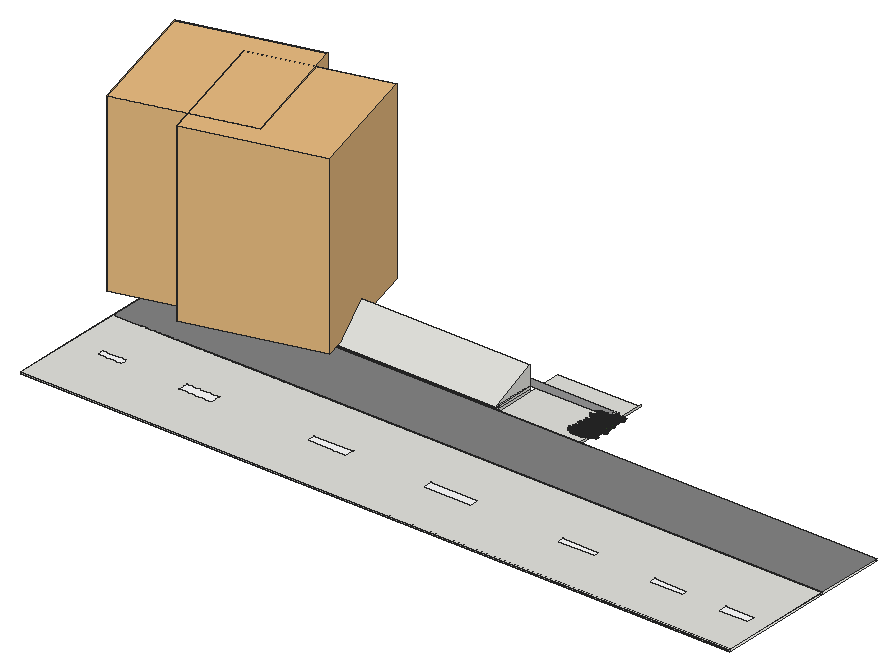
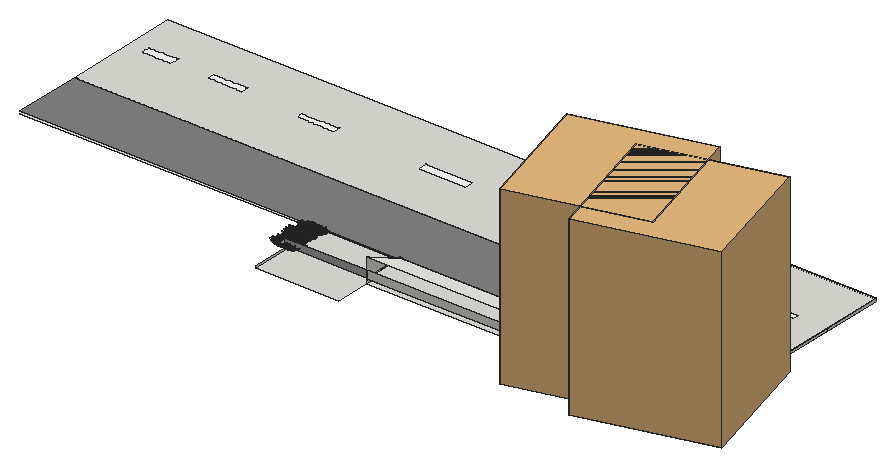
# SketchUp Ruby script. Lengths in inches.
U = 1.inch
M = Sketchup.active_model
def pt(a) = Geom::Point3d.new(a.map { |v| v * U })
def face(e, loops, mat)
  f = e.add_face(loops[0].map { |a| pt(a) })
  loops[1..].each { |l| e.add_face(l.map { |a| pt(a) }).erase! }
  f.material = f.back_material = mat if mat
  f
end
# faces: each face lists its corners as indices into pts; further lists are holes
def faces(e, pts, list, mat = nil) = list.each { |f| face(e, (f[0].is_a?(Array) ? f : [f]).map { |l| l.map { |i| pts[i] } }, mat) }
# xy, xz, yz: faces in a plane at the given z, y or x. An outline is a flat list of corners, or four numbers for a rectangle; further outlines are holes
def ring(l) = l.size == 4 ? [[l[0], l[1]], [l[2], l[1]], [l[2], l[3]], [l[0], l[3]]] : l.each_slice(2).to_a
def flat(e, list, mat, &to3) = list.each { |f| face(e, (f[0].is_a?(Array) ? f : [f]).map { |l| ring(l).map { |u, v| to3.(u, v) } }, mat) }
def xy(e, z, list, mat = nil) = flat(e, list, mat) { |x, y| [x, y, z] }
def xz(e, y, list, mat = nil) = flat(e, list, mat) { |x, z| [x, y, z] }
def yz(e, x, list, mat = nil) = flat(e, list, mat) { |y, z| [x, y, z] }
def lines(e, pts, list) = list.each { |a, b| e.add_line(pt(pts[a]), pt(pts[b])) }
# prism: a flat outline (further loops are holes) pulled along v
def prism(e, loops, v, mat = nil)
  f = face(e, loops, mat); d = Geom::Vector3d.new(v.map { |x| x * U })
  f.pushpull(f.normal.samedirection?(d) ? d.length : -d.length)
end
def box(e, o, s, mat = nil) = prism(e, [[o, [o[0] + s[0], o[1], o[2]], [o[0] + s[0], o[1] + s[1], o[2]], [o[0], o[1] + s[1], o[2]]]], [0, 0, s[2]], mat)
def at(x, y, z, deg = 0) = Geom::Transformation.translation(pt([x, y, z])) * Geom::Transformation.rotation(ORIGIN, Z_AXIS, deg.degrees)
def axes(o, x, y, z) = Geom::Transformation.new([*x, 0, *y, 0, *z, 0, *pt(o).to_a, 1])
def part(name) = M.definitions.add(name)
# library, detail: a bought-in or finely detailed component or shape, given as its bounding box
def library(name, o, s) = part(name).tap { |d| box(d.entities, o, s) }
def detail(e, o, s) = box(e.add_group.entities, o, s)
def put(e, d, t, mat = nil) = e.add_instance(d, t).tap { |i| i.material = mat if mat }
def group(e, t, mat = nil) = e.add_group.tap { |g| g.transformation = t; g.material = mat if mat }.entities
root = M.entities
M.materials.add("Color_3").color = [255, 255, 255]
M.materials.add("Material82").color = [68, 110, 58]
M.materials.add("Material83").color = [48, 90, 38]
M.materials.add("Material84").color = [68, 110, 48]
M.materials.add("Material85").color = [48, 90, 48]
M.materials.add("Material86").color = [58, 110, 58]
M.materials.add("Material87").color = [58, 90, 38]
M.materials.add("Material88").color = [68, 100, 58]
M.materials.add("Material89").color = [48, 100, 38]
M.materials.add("[Color M03]1").color = [170, 170, 170]
M.materials.add("[Tile Grey]1").color = [132, 132, 132]
c1 = library("Palm tree",[-4.09,-4.52,0],[193.52,193.51,258.93])
c2 = part("Palm+Tree")
put(c2.entities,c1,at(25.51,-21.81,0,15))
c3 = library("Group\#612",[0,0,0],[32.91,53.52,103.45])
c4 = part("Untitled (5)")
xy(c4.entities,0,[[[158.81,26.5625,306.06,993.3125],[226.57,518.17,239.57,583.92],[225.28,357.51,237.28,411.51],[222.61,182.28,236.36,226.53],[239.71,931.55,251.46,972.3],[233.64,703.93,242.14,755.18],[240.05,835.03,248.8,880.53],[222.04,66.5,231.29,100.5]]])
xy(c4.entities,0,[[222.04,66.5,231.29,100.5],[222.61,182.28,236.36,226.53],[225.28,357.51,237.28,411.51],[226.57,518.17,239.57,583.92],[233.64,703.93,242.14,755.18],
  [240.05,835.03,248.8,880.53],[239.71,931.55,251.46,972.3]],"Color_3")
c5 = part("grass00")
p = [[-0.6875,0.15,0],[-0.56,0.08,5.52],[-0.04,0.03,2.76],[0.48,-0.02,0],[0.35,-0.02,5.52],[-0.1,-0.14,5.52],
  [-0.12,0.65,8.37],[-0.42,0.65,8.37]]
faces(c5.entities,p,[[0,1,2,3],[3,2,4],[1,5,2],[5,4,2],[1,6,5],[4,5,6],[7,6,1]])
c6 = part("Group16\#1")
put(c6.entities,c5,axes([1.44,-0.61,-0.01],[0.05352,0.12609,0],[-0.10704,0.04543,0.07239],[0.06664,-0.02828,0.11628]),"Material85")
put(c6.entities,c5,axes([0.76,-0.15,-0.01],[0.04676,0.24062,0],[-0.23162,0.04501,0.06642],[0.0652,-0.01267,0.23595]),"Material82")
put(c6.entities,c5,axes([0.79,0.01,-0.01],[-0.00606,0.34651,0],[-0.34381,-0.00602,0.0432],[0.04319,0.00076,0.34386]))
put(c6.entities,c5,axes([1,0.23,-0.01],[-0.07192,0.31144,0],[-0.28722,-0.06632,0.1236],[0.12043,0.02781,0.29478]),"Material84")
put(c6.entities,c5,axes([1.66,0.77,-0.01],[-0.13828,0.29651,0],[-0.21551,-0.1005,0.22471],[0.20365,0.09498,0.23779]),"Material89")
put(c6.entities,c5,axes([0.6875,0.52,-0.01],[-0.18126,0.24051,0],[-0.22746,-0.17142,0.09788],[0.07817,0.05891,0.28481]),"Material84")
put(c6.entities,c5,axes([0.68,0.78,-0.01],[-0.215,0.18688,0],[-0.12385,-0.14248,0.21334],[0.13995,0.16101,0.18878]),"Material82")
put(c6.entities,c5,axes([0.56,1,-0.01],[-0.13756,0.07624,0],[-0.06159,-0.11112,0.0927],[0.04494,0.08108,0.12705]),"Material84")
put(c6.entities,c5,axes([0.2,0.64,-0.01],[-0.23729,0.07254,0],[-0.05711,-0.18681,0.153],[0.04473,0.14632,0.19535]),"Material89")
put(c6.entities,c5,axes([0.0625,0.72,-0.01],[-0.28874,0.02525,0],[-0.02179,-0.24916,0.14647],[0.01276,0.14591,0.25012]),"Material82")
put(c6.entities,c5,axes([-0.08,0.62,-0.01],[-0.34089,-0.04187,0],[0.03255,-0.26504,0.216],[-0.02633,0.21439,0.26703]),"Material89")
put(c6.entities,c5,axes([-0.34,0.98,-0.01],[-0.14314,-0.0493,0],[0.04397,-0.12769,0.06843],[-0.02228,0.0647,0.13505]),"Material89")
put(c6.entities,c5,axes([-0.87,1.45,-0.01],[-0.23488,-0.14114,0],[0.13761,-0.22901,0.06087],[-0.03135,0.05217,0.26717]))
put(c6.entities,c5,axes([-0.72,0.77,-0.01],[-0.14208,-0.13251,0],[0.07209,-0.0773,0.16301],[-0.11118,0.11922,0.1057]),"Material89")
put(c6.entities,c5,axes([-0.62,0.43,-0.01],[-0.14845,-0.21203,0],[0.18654,-0.13061,0.12304],[-0.10079,0.07057,0.22772]),"Material82")
put(c6.entities,c5,axes([-0.68,0.29,-0.01],[-0.13639,-0.32136,0],[0.31723,-0.13464,0.05579],[-0.05136,0.0218,0.34462]),"Material83")
put(c6.entities,c5,axes([-0.64,0.125,-0.01],[-0.0458,-0.23569,0],[0.22124,-0.043,0.08276],[-0.08124,0.01579,0.22538]),"Material86")
put(c6.entities,c5,axes([-1.6,-0.03,-0.01],[0.00576,-0.32897,0],[0.27526,0.00482,0.18018],[-0.18015,-0.00315,0.2753]),"Material84")
put(c6.entities,c5,axes([-1.36,-0.31,-0.01],[0.05718,-0.24765,0],[0.18172,0.04196,0.17267],[-0.16825,-0.03885,0.1865]),"Material89")
put(c6.entities,c5,axes([-1.54,-0.72,-0.01],[0.06537,-0.14017,0],[0.13555,0.06321,0.03939],[-0.0357,-0.01665,0.14956]))
put(c6.entities,c5,axes([-1.19,-0.9,-0.01],[0.09597,-0.12735,0],[0.11214,0.08451,0.07557],[-0.06035,-0.04548,0.14042]),"Material88")
put(c6.entities,c5,axes([-0.47,-0.54,-0.01],[0.11588,-0.10072,0],[0.0618,0.0711,0.12124],[-0.07953,-0.0915,0.0942]))
put(c6.entities,c5,axes([-0.47,-0.84,-0.01],[0.11927,-0.0661,0],[0.06603,0.11913,0.00646],[-0.00313,-0.00565,0.13621]),"Material84")
put(c6.entities,c5,axes([-0.38,-1.24,-0.01],[0.28037,-0.08571,0],[0.0618,0.20215,0.20315],[-0.05939,-0.19428,0.21139]),"Material88")
put(c6.entities,c5,axes([-0.06,-0.66,-0.01],[0.22719,-0.01987,0],[0.01247,0.14255,0.17758],[-0.01547,-0.17691,0.1431]),"Material87")
put(c6.entities,c5,axes([0.11,-0.89,-0.01],[0.14882,0.01828,0],[-0.01058,0.08611,0.12229],[0.01491,-0.12138,0.08676]),"Material85")
put(c6.entities,c5,axes([0.25,-0.72,-0.01],[0.20481,0.07053,0],[-0.06206,0.18022,0.10291],[0.03351,-0.0973,0.1906]),"Material85")
put(c6.entities,c5,axes([0.85,-1.42,-0.01],[0.16481,0.09904,0],[-0.09472,0.15762,0.05616],[0.02893,-0.04814,0.18389]),"Material84")
put(c6.entities,c5,axes([1.01,-1.09,-0.01],[0.21858,0.20385,0],[-0.17495,0.1876,0.15339],[0.10462,-0.11218,0.25652]),"Material89")
put(c6.entities,c5,axes([1.01,-0.71,-0.01],[0.08733,0.12473,0],[-0.06445,0.04512,0.13037],[0.1068,-0.07477,0.07867]),"Material85")
c7 = part("Group15\#1")
put(c7.entities,c6,at(0,0,0))
c8 = part("3darcstudiotree_grass00\#1")
put(c8.entities,c7,at(0,0,0))
xy(root,-42.1875,[[1048.66,1.59,2096.97,172.28],[1048.66,172.28,1248.34,273.41],[1248.34,172.28,1248.34,273.41,1534.73,273.41,1534.73,387.84,1657.41,387.84,1657.41,273.41,2096.97,273.41,2096.97,172.28],[1048.66,273.41,1534.73,335.84]])
xy(root,-39.1875,[[1048.66,1.59,2096.97,172.28]])
xy(root,-38.61,[[1048.66,172.28,2096.97,273.41]],"[Tile Grey]1")
xy(root,-38.0625,[[1048.66,273.41,1164.28,273.53],[1164.28,273.41,1534.73,273.53]])
xy(root,-35.625,[[1248.34,273.41,1534.73,273.53],[1248.34,273.53,1534.73,335.84]])
xy(root,-34.17,[[1164.28,273.41,1248.34,273.53]])
xz(root,1.59,[[1048.66,-42.1875,2096.97,-39.1875]])
xz(root,172.28,[[1048.66,-42.1875,1248.34,-39.1875],[1248.34,-42.1875,2096.97,-39.1875],[1048.66,-39.1875,1248.34,-38.61],[1248.34,-39.1875,2096.97,-38.61]])
xz(root,273.41,[[1048.66,-42.1875,1248.34,-38.61],[1248.34,-42.1875,1534.73,-39.125],[1657.41,-42.1875,1674.99,-39.125],[1248.34,-39.125,1534.73,-38.61],[1534.73,-39.125,1657.41,-38.61],
  [1657.41,-39.125,1674.99,-38.61],[1048.66,-38.61,1534.73,-38.1875],[1534.73,-38.61,1657.41,-38.1875],[1048.66,-38.1875,1534.73,-38.0625],[1164.28,-38.0625,1534.73,-38.0625,1534.73,-35.625,1248.34,-35.625,1248.34,-34.17,1164.28,-34.17]])
xz(root,273.53,[[1048.66,-38.0625,1164.28,-34.17],[1164.28,-38.0625,1164.28,-34.17,1248.34,-34.17,1248.34,-35.625,1534.73,-35.625,1534.73,-38.0625]])
xz(root,335.84,[[1248.34,-35.625,1534.73,-24.25]])
xz(root,335.84,[[1534.73,-34.17,1657.41,-24.25]],"[Color M03]1")
yz(root,1048.66,[[1.59,-42.1875,90.97,-39.1875],[90.97,-42.1875,172.28,-39.1875],[172.28,-42.1875,273.41,-38.61],[273.41,-42.1875,387.84,-42.1875,387.84,-34.17,273.53,-34.17,273.53,-38.0625,273.41,-38.0625],[273.41,-38.0625,273.53,-34.17]])
yz(root,1164.28,[[273.41,-38.0625,273.53,-34.17]])
yz(root,1248.34,[[273.41,-35.625,273.53,-35.57,273.53,-34.17,273.41,-34.17],[273.41,-35.625,273.53,-35.625,273.53,-35.57],[273.53,-35.625,273.53,-35.57,276.53,-34.17,335.84,-34.17,335.84,-35.625],[273.53,-35.57,276.53,-34.17,273.53,-34.17],[276.53,-34.17,335.84,-6.625,335.84,-34.17]])
yz(root,1534.73,[[273.41,-42.1875,335.84,-39.125],[273.41,-39.125,273.41,-38.0625,273.53,-38.0625,273.53,-35.625,335.84,-35.625,335.84,-39.125],[273.41,-38.0625,273.53,-37.86],[273.41,-37.86,273.53,-37.24],[273.41,-37.24,273.53,-35.625],
  [273.41,-35.625,273.41,-34.17,276.53,-34.17],[273.41,-35.625,335.84,-35.625,335.84,-34.17,276.53,-34.17],[276.53,-34.17,335.84,-34.17,335.84,-6.625]])
yz(root,1657.41,[[273.41,-42.1875,387.84,-39.125],[335.84,-34.17,341.03,-27.66]])
p = [[1248.34,335.84,-6.625],[1248.34,276.53,-34.17],[1248.34,273.53,-35.57],[1248.34,273.41,-35.625],[1534.73,273.41,-35.625],[1534.73,276.53,-34.17],
  [1534.73,335.84,-6.625]]
faces(root,p,[[0,1,2,3,4,5,6]])
put(root,c2,at(990.76,232.43,-34.17))
put(root,c3,axes([1115.7,235.4,-34.17],[1.13014,0.75656,0],[-0.75656,1.13014,0],[0,0,1.36]))
put(root,c2,at(1097.7,226.62,-34.17))
put(root,c4,axes([1020.1875,358.09,-38.61],[0,-1.17,0],[1.0847,0,0],[0,0,1]))
put(root,c8,axes([1645.78,299.125,-34.17],[-1.33725,-1.41841,0],[4.13991,-0.60704,-0.02925],[0.14115,-0.0207,1.7044]))
put(root,c8,axes([1645.82,287.75,-34.17],[-4.40805,-0.66258,0],[1.20213,-1.24385,-0.04688],[0.1049,-0.10854,1.58936]))
put(root,c8,axes([1645.93,289.38,-34.17],[-4.593,-0.45536,0],[0.84159,-1.32024,-0.02201],[0.02791,-0.04378,1.34565]))
put(root,c8,axes([1645.18,338.56,-34.17],[2.83648,-1.2359,0],[3.15131,1.12486,-0.01132],[0.04822,0.01721,1.83032]))
put(root,c8,axes([1646.2,324.1,-34.17],[-1.4633,-1.68853,0],[3.81957,-0.51482,-0.03013],[0.1448,-0.01952,1.53631]))
put(root,c8,axes([1644.93,281.03,-34.17],[3.65261,0,0],[0,1.44049,0],[0,0,1]))
put(root,c8,axes([1645.16,323.0625,-34.17],[3.25905,0.69762,0],[-2.04099,1.48295,-0.01651],[-0.04447,0.03231,1.81134]))
put(root,c8,axes([1645.93,301.17,-34.17],[-1.85538,1.37845,0],[-3.32658,-0.69639,-0.02935],[-0.1215,-0.02544,1.32321]))
put(root,c8,axes([1645.82,333.36,-34.17],[-2.16254,1.46376,0],[-3.92939,-0.90288,-0.00219],[-0.00913,-0.0021,1.64693]))
put(root,c8,axes([1645.98,292.54,-34.17],[3.24585,-0.20669,0],[0.57348,1.40067,-0.03713],[0.03058,0.07468,1.39317]))
put(root,c8,axes([1646.36,320.21,-34.17],[3.32132,-0.19382,0],[0.6507,1.73421,-0.00326],[0.00271,0.00722,1.88794]))
put(root,c8,axes([1646.24,283.13,-34.17],[1.50682,1.6341,0],[-3.24176,0.46492,-0.03897],[-0.21712,0.03114,1.53286]))
put(root,c8,axes([1648.33,326.94,-34.17],[-4.71763,0.13616,0],[-0.3116,-1.67918,-0.0067],[-0.002,-0.01078,1.30916]))
put(root,c8,axes([1648.23,333.39,-34.17],[0.36596,-1.66077,0],[4.11633,0.14107,-0.03115],[0.15736,0.00539,1.5702]))
put(root,c8,axes([1648.77,328.95,-34.17],[1.0844,-1.46677,0],[3.4842,0.40063,-0.01207],[0.07085,0.00815,1.66287]))
put(root,c8,axes([1649,283.72,-34.17],[2.27608,-1.0007,0],[3.35316,1.18618,-0.03873],[0.1622,0.05738,1.89965]))
put(root,c8,axes([1649.48,313.58,-34.17],[-3.59463,0.44793,0],[-1.16817,-1.45801,-0.02199],[-0.03431,-0.04283,1.50537]))
put(root,c8,axes([1649.46,309.39,-34.17],[2.73821,-1.25836,0],[3.57659,1.21044,-0.00643],[0.02336,0.00791,1.6911]))
put(root,c8,axes([1648.61,339.7,-34.17],[4.22455,0.00563,0],[-0.01154,1.34671,-0.00416],[-0.00007,0.00858,1.3392]))
put(root,c8,axes([1648.76,330.83,-34.17],[-0.387,1.5813,0],[-4.71042,-0.17929,-0.01578],[-0.06068,-0.00231,1.37044]))
put(root,c8,axes([1648.82,298.98,-34.17],[0.67723,1.39261,0],[-4.43088,0.33513,-0.00068],[-0.00322,0.00024,1.62852]))
put(root,c8,axes([1650.27,317.53,-34.17],[1.58844,-1.66939,0],[3.21642,0.47599,-0.02337],[0.14197,0.02101,1.67088]))
put(root,c8,axes([1650.63,287.01,-34.17],[-3.67612,0.09043,0],[-0.28445,-1.79854,-0.0193],[-0.00469,-0.02963,1.33558]))
put(root,c8,axes([1649.59,285.78,-34.17],[0.19969,1.44757,0],[-3.37153,0.07234,-0.03311],[-0.18886,0.00405,1.44579]))
put(root,c8,axes([1650.98,335.77,-34.17],[0.06282,-1.34984,0],[3.50326,0.02536,-0.01436],[0.0861,0.00062,1.57494]))
put(root,c8,axes([1650.16,289.01,-34.17],[-2.51102,1.11498,0],[-3.04783,-1.06754,-0.01682],[-0.06435,-0.02254,1.56312]))
put(root,c8,axes([1651.08,322.91,-34.17],[-3.50605,0.34582,0],[-0.87343,-1.37724,-0.00789],[-0.01222,-0.01927,1.7222]))
put(root,c8,axes([1649.97,292.59,-34.17],[4.50029,0.14913,0],[-0.32235,1.51291,-0.00911],[-0.00515,0.02417,1.94776]))
put(root,c8,axes([1651.2,316.28,-34.17],[-3.11045,1.07931,0],[-2.57078,-1.15227,-0.02195],[-0.09054,-0.04058,1.82186]))
put(root,c8,axes([1651.67,321.04,-34.17],[2.67895,-1.42027,0],[3.76202,1.10364,-0.01386],[0.04132,0.01212,1.30579]))
put(root,c8,axes([1652.24,305.28,-34.17],[-4.02887,-0.32689,0],[0.86941,-1.66657,-0.02294],[0.02463,-0.04722,1.72347]))
put(root,c8,axes([1651.25,300.74,-34.17],[3.37179,-0.80655,0],[2.39395,1.55652,-0.03972],[0.09789,0.06365,1.6444]))
put(root,c8,axes([1650.47,324.46,-34.17],[3.19117,1.02249,0],[-2.28557,1.10943,-0.0068],[-0.02189,0.01063,1.38619]))
put(root,c8,axes([1650.56,307.12,-34.17],[0.53207,1.56479,0],[-4.35061,0.23008,-0.0098],[-0.05087,0.00269,1.72283]))
put(root,c8,axes([1650.68,311.99,-34.17],[3.6725,0.99677,0],[-2.44181,1.39924,-0.05897],[-0.19798,0.11345,1.91169]))
put(root,c8,axes([1651.48,338.53,-34.17],[-1.969,1.11609,0],[-3.42444,-0.93961,-0.02835],[-0.10891,-0.02988,1.46355]))
put(root,c8,axes([1651.98,295.5,-34.17],[-3.28336,1.15138,0],[-2.69769,-1.19648,-0.01814],[-0.06877,-0.0305,1.73642]))
put(root,c8,axes([1652.11,303.28,-34.17],[-2.75837,1.17724,0],[-3.35186,-1.22148,-0.01856],[-0.07358,-0.02681,1.84646]))
put(root,c8,axes([1651.72,281.08,-34.17],[4.03336,-0.1179,0],[0.28483,1.51556,-0.02045],[0.00943,0.05018,1.8024]))
put(root,c8,axes([1652.2,294.67,-34.17],[1.54692,1.35045,0],[-3.5946,0.6404,-0.01637],[-0.06936,0.01236,1.37485]))
put(root,c8,axes([1653.77,328.81,-34.17],[-1.02138,-1.60708,0],[3.36091,-0.33222,-0.0349],[0.24018,-0.02374,1.84282]))
put(root,c8,axes([1654.79,289.78,-34.17],[-4.39876,-0.08421,0],[0.22064,-1.79246,-0.01036],[0.00206,-0.01674,1.39846]))
put(root,c8,axes([1655.125,316.47,-34.17],[-2.27298,-1.15312,0],[2.90139,-0.88948,-0.04864],[0.26323,-0.0807,1.88819]))
put(root,c8,axes([1655.11,298.2,-34.17],[-0.27323,-1.39515,0],[4.04907,-0.12333,-0.04603],[0.24308,-0.0074,1.61216]))
put(root,c8,axes([1654.6,336.26,-34.17],[-3.30373,1.03648,0],[-2.84639,-1.41107,-0.00639],[-0.01873,-0.00928,1.6128]))
put(root,c8,axes([1655.6,318.86,-34.17],[-4.23108,-0.20575,0],[0.45076,-1.44167,-0.03319],[0.02288,-0.07317,1.55524]))
put(root,c8,axes([1655.91,332.78,-34.17],[-1.34868,-1.52366,0],[4.27,-0.58784,-0.05387],[0.21958,-0.03023,1.46363]))
put(root,c8,axes([1654.57,307.0625,-34.17],[3.56541,-0.13016,0],[0.37676,1.60514,-0.05657],[0.02546,0.10845,1.49576]))
put(root,c8,axes([1655.38,309.03,-34.17],[-3.05652,0.90078,0],[-1.97442,-1.04198,-0.01872],[-0.07362,-0.03885,1.62421]))
put(root,c8,axes([1655.57,285.95,-34.17],[-3.18956,0.31713,0],[-1.10467,-1.728,-0.01943],[-0.01876,-0.02934,1.33771]))
put(root,c8,axes([1656.13,322.01,-34.17],[-3.13974,-0.75675,0],[2.02292,-1.30536,-0.04274],[0.1274,-0.08221,1.66217]))
put(root,c8,axes([1656.26,326.61,-34.17],[-4.11825,0.06325,0],[-0.12995,-1.31605,-0.00954],[-0.0021,-0.02124,1.41434]))
put(root,c8,axes([1655.38,324.39,-34.17],[-0.62058,1.51993,0],[-3.60511,-0.22893,-0.03829],[-0.23497,-0.01492,1.70109]))
put(root,c8,axes([1656.78,313.68,-34.17],[-0.89443,-1.66932,0],[4.23179,-0.35265,-0.02196],[0.11928,-0.00994,1.79942]))
put(root,c8,axes([1655,304.39,-34.17],[2.80483,0.78712,0],[-2.29694,1.27299,-0.00585],[-0.01927,0.01068,1.68777]))
put(root,c8,axes([1656.43,292.6,-34.17],[1.02165,-1.42104,0],[3.23224,0.36142,-0.01712],[0.09227,0.01032,1.41054]))
put(root,c8,axes([1657.18,303.62,-34.17],[-4.34806,-0.2749,0],[0.62437,-1.53594,-0.05495],[0.04724,-0.1162,1.60563]))
put(root,c8,axes([1656.82,337.26,-34.17],[1.68936,-1.29831,0],[3.68445,0.74564,-0.0206],[0.10358,0.02096,1.75423]))
put(root,c8,axes([1657.04,311.5625,-34.17],[0.80832,-1.39105,0],[3.86121,0.34896,-0.01662],[0.09893,0.00894,1.81323]))
put(root,c8,axes([1655.86,301.28,-34.17],[1.77276,1.31188,0],[-3.2596,0.68507,-0.05193],[-0.30681,0.06448,1.85357]))
put(root,c8,axes([1657.41,319.51,-34.17],[0.5287,-1.47174,0],[3.5141,0.19634,-0.02485],[0.18259,0.0102,1.97391]))
put(root,c8,axes([1657.29,282.72,-34.17],[3.14916,-0.41283,0],[1.21857,1.44573,-0.00205],[0.00401,0.00476,1.79239]))
put(root,c8,axes([1657.375,287.375,-34.17],[-1.68906,1.71794,0],[-3.99186,-0.61041,-0.03012],[-0.15949,-0.02439,1.82227]))
put(root,c8,axes([1657.24,330.84,-34.17],[2.62983,0.98737,0],[-2.70679,1.12128,-0.04733],[-0.14621,0.06057,1.31836]))
put(root,c8,axes([1657.59,293.36,-34.17],[2.45025,1.521,0],[-3.17244,0.79485,-0.05376],[-0.27331,0.06848,1.69687]))
put(root,c8,axes([1657.67,296.36,-34.17],[3.99404,0.60234,0],[-1.558,1.60676,-0.01506],[-0.02517,0.02596,1.52965]))
put(root,c8,axes([1659.51,289.58,-34.17],[-3.18903,-1.00454,0],[2.15912,-1.06605,-0.04095],[0.17363,-0.08573,1.76156]))
put(root,c8,axes([1659.59,291.41,-34.17],[1.91072,-1.36379,0],[2.93743,0.64007,-0.00396],[0.02678,0.00583,1.94458]))
put(root,c8,axes([1659.68,294.55,-34.17],[-3.96013,0.90558,0],[-1.84066,-1.25189,-0.01457],[-0.03554,-0.02417,1.33777]))
put(root,c8,axes([1659.89,322.82,-34.17],[-1.43633,1.59136,0],[-3.83282,-0.53804,-0.05045],[-0.25445,-0.03572,1.63245]))
put(root,c8,axes([1661.32,302.28,-34.17],[-1.0696,-1.4156,0],[4.38412,-0.5152,-0.01047],[0.05162,-0.00607,1.7643]))
put(root,c8,axes([1659.51,324.46,-34.17],[1.80901,1.52238,0],[-3.47581,0.64237,-0.0367],[-0.2302,0.04254,1.99296]))
put(root,c8,axes([1661.02,283.32,-34.17],[-3.28831,-0.06152,0],[0.17407,-1.44709,-0.03298],[0.01066,-0.08861,1.87797]))
put(root,c8,axes([1661.17,333.28,-34.17],[-0.39059,-1.54022,0],[4.16557,-0.16429,-0.04439],[0.19629,-0.00774,1.39437]))
put(root,c8,axes([1661.18,306.79,-34.17],[-3.41271,-0.33865,0],[0.85241,-1.336,-0.02412],[0.03639,-0.05703,1.61843]))
put(root,c8,axes([1661.57,313.34,-34.17],[-2.93694,-0.59609,0],[2.12271,-1.62662,-0.00712],[0.01544,-0.01183,1.64666]))
put(root,c8,axes([1661.05,315.2,-34.17],[-3.29904,0.80499,0],[-2.22234,-1.41651,-0.03047],[-0.07031,-0.04481,1.38852]))
put(root,c8,axes([1660.4,331.79,-34.17],[4.14707,-0.51237,0],[1.30496,1.64274,-0.0458],[0.07431,0.09355,1.7756]))
put(root,c8,axes([1660.07,286.73,-34.17],[3.27777,1.34463,0],[-2.52219,0.95624,-0.03508],[-0.15429,0.0585,1.59982]))
put(root,c8,axes([1661.2,284.89,-34.17],[2.26051,-1.27757,0],[3.2134,0.8843,-0.05108],[0.25562,0.07035,1.79238]))
put(root,c8,axes([1660.81,320.12,-34.17],[-1.59446,1.31407,0],[-3.90941,-0.73777,-0.03408],[-0.12847,-0.02424,1.35762]))
put(root,c8,axes([1662.24,317.48,-34.17],[-0.30604,-1.61832,0],[4.50612,-0.13253,-0.02024],[0.10989,-0.00323,1.84439]))
put(root,c8,axes([1661.41,309.01,-34.17],[3.41243,-1.19241,0],[2.8473,1.26731,-0.01442],[0.05672,0.02524,1.90876]))
put(root,c8,axes([1661.08,304.59,-34.17],[-1.88838,1.28179,0],[-3.89061,-0.89146,-0.00809],[-0.03969,-0.00909,1.91363]))
put(root,c8,axes([1661.68,335.43,-34.17],[2.99246,-1.30733,0],[3.43775,1.22386,-0.0538],[0.15792,0.05622,1.37259]))
put(root,c8,axes([1661.49,299.03,-34.17],[3.20139,-0.30461,0],[0.92111,1.5056,-0.01591],[0.01676,0.0274,1.32206]))
put(root,c8,axes([1662.82,328.74,-34.17],[0.73171,-1.70112,0],[4.49029,0.30039,-0.00997],[0.04273,0.00286,1.48373]))
put(root,c8,axes([1662.2,300.2,-34.17],[-2.68631,1.22242,0],[-2.89186,-0.98838,-0.03703],[-0.15503,-0.05299,1.58908]))
put(root,c8,axes([1661.43,326.42,-34.17],[1.0764,1.4346,0],[-4.21811,0.49224,-0.04809],[-0.1912,0.02231,1.36712]))
put(root,c8,axes([1661.56,295.86,-34.17],[4.09217,0.10074,0],[-0.26997,1.70555,-0.00965],[-0.00291,0.01837,1.57035]))
put(root,c8,axes([1661.69,337.93,-34.17],[1.32449,1.52251,0],[-4.11933,0.55735,-0.02597],[-0.14801,0.02003,1.96681]))
put(root,c8,axes([1663,311.93,-34.17],[3.3532,-0.49547,0],[1.21799,1.28203,-0.02122],[0.05381,0.05664,1.88089]))
put(root,c8,axes([1664.97,324.53,-34.17],[-3.17181,-0.36437,0],[1.29907,-1.75875,-0.03129],[0.04635,-0.06275,1.8441]))
put(root,c8,axes([1665.14,311.13,-34.17],[-3.51166,-0.15133,0],[0.49376,-1.78204,-0.01667],[0.00952,-0.03434,1.79039]))
put(root,c8,axes([1665.59,300.8,-34.17],[-4.25679,0.36903,0],[-0.81289,-1.45836,-0.01858],[-0.01888,-0.03387,1.34303]))
put(root,c8,axes([1666.06,287.33,-34.17],[-2.72023,-1.01034,0],[2.91962,-1.22258,-0.03536],[0.13675,-0.05727,1.8008]))
put(root,c8,axes([1665.42,337.87,-34.17],[-2.05483,1.19866,0],[-3.00093,-0.80011,-0.04556],[-0.27207,-0.07254,1.95702]))
put(root,c8,axes([1665.02,305.8,-34.17],[-0.97742,1.77445,0],[-3.78925,-0.32463,-0.03052],[-0.14263,-0.01222,1.38983]))
put(root,c8,axes([1664.99,315.5625,-34.17],[-0.8481,1.42544,0],[-3.97449,-0.36778,-0.03302],[-0.15824,-0.01464,1.5061]))
